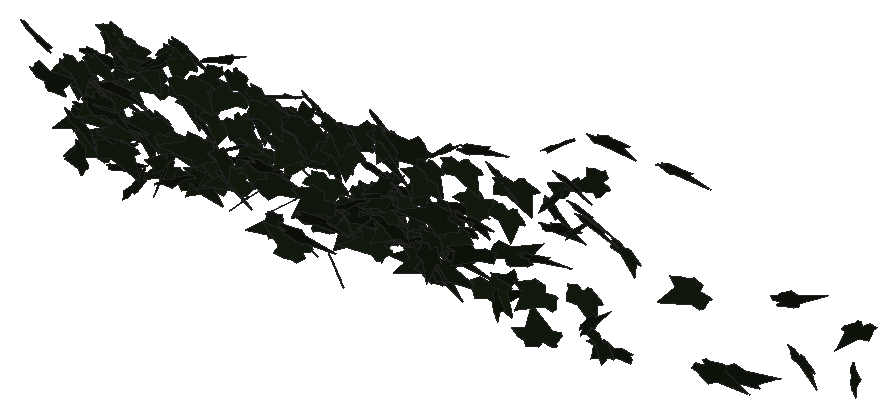
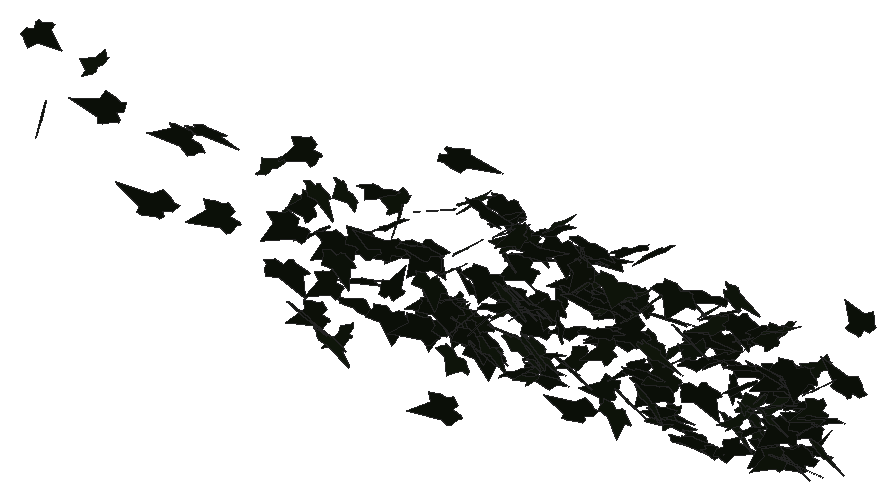
# SketchUp Ruby script. Lengths in millimetres.
U = 1.mm
M = Sketchup.active_model
def pt(a) = Geom::Point3d.new(a.map { |v| v * U })
def face(e, loops, mat)
  f = e.add_face(loops[0].map { |a| pt(a) })
  loops[1..].each { |l| e.add_face(l.map { |a| pt(a) }).erase! }
  f.material = f.back_material = mat if mat
  f
end
# faces: each face lists its corners as indices into pts; further lists are holes
def faces(e, pts, list, mat = nil) = list.each { |f| face(e, (f[0].is_a?(Array) ? f : [f]).map { |l| l.map { |i| pts[i] } }, mat) }
# xy, xz, yz: faces in a plane at the given z, y or x. An outline is a flat list of corners, or four numbers for a rectangle; further outlines are holes
def ring(l) = l.size == 4 ? [[l[0], l[1]], [l[2], l[1]], [l[2], l[3]], [l[0], l[3]]] : l.each_slice(2).to_a
def flat(e, list, mat, &to3) = list.each { |f| face(e, (f[0].is_a?(Array) ? f : [f]).map { |l| ring(l).map { |u, v| to3.(u, v) } }, mat) }
def xy(e, z, list, mat = nil) = flat(e, list, mat) { |x, y| [x, y, z] }
def xz(e, y, list, mat = nil) = flat(e, list, mat) { |x, z| [x, y, z] }
def yz(e, x, list, mat = nil) = flat(e, list, mat) { |y, z| [x, y, z] }
def lines(e, pts, list) = list.each { |a, b| e.add_line(pt(pts[a]), pt(pts[b])) }
# prism: a flat outline (further loops are holes) pulled along v
def prism(e, loops, v, mat = nil)
  f = face(e, loops, mat); d = Geom::Vector3d.new(v.map { |x| x * U })
  f.pushpull(f.normal.samedirection?(d) ? d.length : -d.length)
end
def box(e, o, s, mat = nil) = prism(e, [[o, [o[0] + s[0], o[1], o[2]], [o[0] + s[0], o[1] + s[1], o[2]], [o[0], o[1] + s[1], o[2]]]], [0, 0, s[2]], mat)
def at(x, y, z, deg = 0) = Geom::Transformation.translation(pt([x, y, z])) * Geom::Transformation.rotation(ORIGIN, Z_AXIS, deg.degrees)
def axes(o, x, y, z) = Geom::Transformation.new([*x, 0, *y, 0, *z, 0, *pt(o).to_a, 1])
def part(name) = M.definitions.add(name)
# library, detail: a bought-in or finely detailed component or shape, given as its bounding box
def library(name, o, s) = part(name).tap { |d| box(d.entities, o, s) }
def detail(e, o, s) = box(e.add_group.entities, o, s)
def put(e, d, t, mat = nil) = e.add_instance(d, t).tap { |i| i.material = mat if mat }
def group(e, t, mat = nil) = e.add_group.tap { |g| g.transformation = t; g.material = mat if mat }.entities
root = M.entities
M.materials.add("efeu1").color = [18, 25, 13]
c1 = part("ivyleaf_9")
p = [[39.1,54.8,31.7],[34.5,51.8,30.2],[-5.3,25.2,17.3],[-17.9,28.3,20.9],[-21.6,21.7,17],[-20.2,4.3,5.3],
  [-22.9,-0.3,2.5],[-17.1,-4,-0.6],[-2,-2.1,-1.2],[-0.7,-15.4,-10.1],[16.6,-22.3,-16.7],[21.1,-15.1,-12.5],
  [32.7,-10.7,-11],[46.1,-1.8,-6.6],[30.8,11.2,3.8]]
faces(c1.entities,p,[[0,1,2,3,4,5,6,7,8,9,10,11,12,13,14]],"efeu1")
put(root,c1,axes([6987.3,575.4,5164.4],[-1.35128,-1.10406,-0.33576],[0.69221,0.16003,-1.29534],[2.08434,-0.76891,0.21251]))
put(root,c1,axes([7044.1,521.7,5017.1],[-1.94294,0.95691,-0.16624],[0.20085,-0.13047,-1.39906],[-1.83753,-1.02607,0.02286]))
put(root,c1,axes([6987.6,400.2,5195.8],[-0.31285,0.13905,1.47625],[1.73968,-1.15999,0.21104],[2.22203,0.92777,0.04261]))
put(root,c1,axes([6992.9,326.4,5410.5],[-0.05139,-0.57991,1.37103],[1.05785,-1.27601,-0.52878],[2.62827,0.50224,0.23963]))
put(root,c1,axes([7007,583.9,5129],[0.31005,-1.35705,-0.09852],[-0.02649,0.09755,-1.36679],[2.5894,0.16349,-0.00219]))
put(root,c1,axes([6997.3,554.2,5179.8],[2.301,-0.69536,-0.09625],[-0.09394,0.10701,-1.39306],[1.33272,1.20811,0.06799]))
put(root,c1,axes([7043.8,504.4,5234.5],[-0.08437,-1.39838,0.16525],[-0.01937,-0.16501,-1.39908],[2.67985,-0.04522,-0.00491]))
put(root,c1,axes([7121.3,630.5,4983.1],[-2.28537,0.3892,0.4893],[-1.08791,-0.25428,-1.20059],[-0.48198,-1.27149,0.38988]))
put(root,c1,axes([7082.3,509.9,5078.4],[2.60564,0.29321,0.06626],[0.11968,0.0228,-1.4001],[-0.55946,1.3705,0.00911]))
put(root,c1,axes([7123.6,438.2,4916],[-0.35528,-0.20118,1.47783],[-1.22938,-1.33152,-0.26286],[2.55851,-0.66774,0.07891]))
put(root,c1,axes([7124.9,527.5,5287.4],[2.20419,0.45956,-0.79965],[-1.42967,-0.27475,-1.24586],[-1.01844,1.38031,0.01825]))
put(root,c1,axes([7153.9,497.5,4953.7],[-2.16775,-0.51688,0.6399],[-0.98134,-0.40294,-1.24328],[1.21979,-1.24275,0.13696]))
put(root,c1,axes([7096.2,619.4,5099.9],[2.58102,0.04148,-0.09359],[-0.17912,0.01609,-1.35665],[-0.07663,1.35928,0.01892]))
put(root,c1,axes([7107.5,520.1,5271.7],[1.0316,-1.16959,-0.59984],[-0.29748,0.58688,-1.28557],[2.48389,0.55604,0.09516]))
put(root,c1,axes([7149.5,508.2,5128.5],[-1.49282,-0.91359,0.64291],[-0.64363,-0.55451,-1.20057],[2.02635,-0.84917,0.0923]))
put(root,c1,axes([7168.1,558.9,4955.3],[-2.43955,0.46933,-0.21974],[0.37712,-0.09783,-1.36483],[-0.91134,-1.29683,0.02343]))
put(root,c1,axes([7090.1,540.8,4932.8],[0.54196,-0.25496,1.34292],[2.49688,-0.33411,-0.34163],[0.73031,1.3315,0.17142]))
put(root,c1,axes([7188.4,603.3,5117.5],[-1.42232,1.13045,0.23543],[-0.57317,0.07991,-1.33969],[-2.12158,-0.77945,0.2041]))
put(root,c1,axes([7120.3,626.1,4985.6],[2.35985,-0.43864,-0.32699],[-0.41444,0.34741,-1.29177],[0.95523,1.23437,0.24737]))
put(root,c1,axes([7145,596.4,5170.3],[1.45055,-1.13108,-0.30205],[0.0355,0.3721,-1.34635],[2.22782,0.73052,0.21812]))
put(root,c1,axes([7188.7,595.2,5147.3],[-1.44717,-1.12504,0.32421],[0.05347,-0.404,-1.33604],[2.22767,-0.72117,0.24268]))
put(root,c1,axes([7251.2,579.9,5274.8],[-2.61515,-0.03381,-0.1199],[0.23381,-0.14782,-1.36626],[0.03927,-1.37136,0.15023]))
put(root,c1,axes([7226.7,521.5,5401.1],[-1.51726,-0.92919,0.73564],[0.01191,-0.88988,-1.11723],[2.25553,-0.62036,0.50075]))
put(root,c1,axes([7189.6,489.2,5210.3],[2.76874,0.05186,0.25804],[0.49107,0.00505,-1.4557],[-0.09886,1.47748,-0.00409]))
put(root,c1,axes([7203.1,490.7,5399],[1.15331,-1.28618,-0.12622],[-0.07951,0.11984,-1.42172],[2.45833,0.60728,0.01323]))
put(root,c1,axes([7202.6,303.9,5157.4],[0.75456,-1.30208,0.61517],[0.46064,-0.56873,-1.35977],[2.70177,0.46061,0.06003]))
put(root,c1,axes([7201.2,411.6,5187.7],[-0.01399,-0.12223,-1.45499],[2.65777,0.42429,-0.0427],[0.81147,-1.39177,0.11476]))
put(root,c1,axes([7218.5,528.6,5381.5],[1.75038,-1.05899,0.26601],[0.27644,-0.22605,-1.4021],[2.05961,0.93033,-0.03788]))
put(root,c1,axes([7240.1,494.7,4909.3],[2.00993,0.74421,0.40226],[0.63052,0.22819,-1.29195],[-1.48144,1.10682,-0.00411]))
put(root,c1,axes([7252.6,584.9,5037.9],[-0.08734,-1.29505,-0.4348],[0.28474,0.42767,-1.28959],[2.58431,-0.09089,0.12739]))
put(root,c1,axes([7235.4,424,5135.1],[1.33394,-0.52509,1.12204],[1.82035,-0.58995,-0.87355],[1.49842,1.18414,0.06234]))
put(root,c1,axes([7280.5,491,5377.2],[0.04498,-1.06706,-1.07303],[-0.12078,1.07152,-1.06695],[2.87754,0.06165,-0.02801]))
put(root,c1,axes([7335.9,532.3,5056.2],[-1.16153,1.25574,0.27902],[-0.18578,0.26274,-1.39594],[-2.44115,-0.61749,-0.02653]))
put(root,c1,axes([7332.5,421.3,5106.3],[-0.90991,-0.47412,1.20223],[-1.56419,-0.87769,-0.67297],[1.89811,-0.95057,0.02174]))
put(root,c1,axes([7303.3,520.3,5101.6],[1.35793,-0.75192,-0.96683],[-0.88241,0.86984,-1.01865],[2.15758,0.82899,0.19189]))
put(root,c1,axes([7358,575.3,5238.1],[-2.17136,-0.2832,0.78427],[-1.1956,-0.58206,-1.12405],[1.04353,-1.25616,0.34404]))
put(root,c1,axes([7297.9,619.4,5065.5],[1.10209,-1.24001,-0.0136],[0.2012,0.06432,-1.36302],[2.35153,0.57565,0.123]))
put(root,c1,axes([7308.9,378.5,5059.4],[-0.94605,-0.56739,-1.25746],[2.0907,0.64572,-0.72562],[1.58822,-1.188,0.20617]))
put(root,c1,axes([7365.8,410.2,4886.1],[-1.30624,1.03083,-0.83423],[-0.99321,0.65359,1.23697],[2.3202,0.86013,0.05985]))
put(root,c1,axes([7326.4,511.8,5341],[0.0657,-1.43734,-0.0753],[0.59265,0.081,-1.40331],[2.67443,0.01736,0.31282]))
put(root,c1,axes([7343.6,509.1,5055],[-0.35681,-1.10272,0.87642],[0.44942,-0.89624,-1.07714],[2.64287,0.00353,0.30149]))
put(root,c1,axes([7392.4,585.4,4912.1],[-0.41198,-0.18922,-1.32688],[0.40946,-1.33155,0.15479],[-2.51779,-0.18558,0.24229]))
put(root,c1,axes([7407.9,497.9,5376.7],[0.42589,1.27383,-0.53827],[-0.07165,-0.53946,-1.2923],[-2.63094,0.2209,-0.05194]))
put(root,c1,axes([7426.8,515.5,4974],[-1.04629,1.19055,0.39748],[-0.30552,0.36368,-1.31134],[-2.36919,-0.57267,-0.00643]))
put(root,c1,axes([7391,501.5,5116.7],[-0.05299,-1.40594,-0.24864],[-0.03429,0.24901,-1.40603],[2.71708,-0.02427,-0.0226]))
put(root,c1,axes([7411.5,452.9,5162.2],[-1.55732,-0.68227,-0.87434],[1.59409,0.33202,-1.04295],[1.38348,-1.15056,0.21751]))
put(root,c1,axes([7404.6,599.3,5399.3],[1.86942,-0.96205,-0.2297],[0.12829,0.38808,-1.33715],[1.87806,0.93111,0.31998]))
put(root,c1,axes([7476.3,453.8,5439.4],[-1.74129,0.72344,-0.81171],[0.68212,-0.80089,-1.11779],[-1.95371,-0.92441,0.33319]))
put(root,c1,axes([7459.7,545.7,5395.9],[-0.83055,-1.35508,0.15136],[0.02238,-0.16266,-1.42233],[2.59494,-0.43231,0.06072]))
put(root,c1,axes([7533.7,557.8,5079.8],[0.24493,1.19937,-0.75286],[-0.55996,-0.71682,-1.19225],[-2.63628,0.26369,0.18329]))
put(root,c1,axes([7472.1,595.4,4906],[-0.28252,-0.47476,-1.3209],[2.29902,0.63324,-0.36335],[1.36046,-1.16869,0.33972]))
put(root,c1,axes([7511.1,595.5,5218.2],[-0.96129,-1.29081,-0.17502],[0.07123,0.17326,-1.38583],[2.47812,-0.5057,-0.02806]))
put(root,c1,axes([7519,395,5034.2],[-0.87839,0.45942,-1.23349],[1.69188,-0.85518,-0.65114],[-1.84748,-1.00158,-0.00983]))
put(root,c1,axes([7549.3,623,4908.6],[-2.37495,-0.53442,0.11195],[-0.19758,-0.04195,-1.35749],[1.02022,-1.25218,-0.0023]))
put(root,c1,axes([7527,407,5152.7],[0.42178,-1.04534,-0.88327],[-0.00579,0.8944,-1.05927],[2.6046,0.17126,0.14068]))
put(root,c1,axes([7551.3,447.9,5342.2],[0.33698,-1.42826,0.03133],[-0.02925,-0.03347,-1.43906],[2.71876,0.17667,-0.01937]))
put(root,c1,axes([7610.2,568,5286.8],[-2.27222,0.72043,-0.06653],[0.10954,-0.0334,-1.39442],[-1.3726,-1.19528,-0.00114]))
put(root,c1,axes([7614.3,622.8,4951.6],[-2.50126,-0.3388,0.11687],[-0.15696,-0.14642,-1.35182],[0.66379,-1.31128,0.12075]))
put(root,c1,axes([7575.5,523.6,5182.5],[0.60353,-1.16478,0.83285],[0.52107,-0.78797,-1.20626],[2.67492,0.4163,0.04706]))
put(root,c1,axes([7583,439,5380.6],[-0.49082,-0.96763,-0.97719],[1.34928,0.75838,-0.93807],[2.24271,-0.66803,0.35051]))
put(root,c1,axes([7617.8,561.2,5435.4],[1.49983,1.18306,0.22995],[0.03781,0.26195,-1.41582],[-2.29343,0.778,0.12703]))
put(root,c1,axes([7609.4,581.9,5173.5],[-0.72766,-1.23702,0.49471],[0.00106,-0.51483,-1.28689],[2.53559,-0.35479,0.14251]))
put(root,c1,axes([7663.6,493.3,5399.4],[-1.98425,0.98196,0.09227],[-0.13384,0.05992,-1.43221],[-1.87232,-1.04495,0.00459]))
put(root,c1,axes([7689.1,399,5157.3],[-1.81893,0.01019,1.01738],[-1.9363,0.00189,-0.95576],[-0.0159,-1.39587,0.00613]))
put(root,c1,axes([7666.6,255.1,5106.8],[0.75187,1.35802,-0.05307],[-0.03201,-0.05038,-1.41432],[-2.58637,0.39541,0.00208]))
put(root,c1,axes([7696.1,604.9,4957.4],[-2.09753,-0.34591,0.71878],[-1.32226,-0.18611,-1.15483],[0.74596,-1.30255,-0.02588]))
put(root,c1,axes([7621.7,590,4953.5],[1.7044,-1.06528,0.12002],[0.1563,-0.08776,-1.39168],[2.03427,0.89928,0.00637]))
put(root,c1,axes([7673.8,565.5,5318.7],[-2.41131,-0.65815,-0.08821],[0.51998,-0.34349,-1.36145],[1.15187,-1.22271,0.42994]))
put(root,c1,axes([7660.7,553.6,5089.7],[1.46282,0.64431,0.97009],[0.94644,0.86944,-0.97147],[-2.00417,0.88086,0.2493]))
put(root,c1,axes([7715.4,625.2,5022.3],[-0.8237,1.19139,0.5005],[-0.27125,0.4806,-1.26725],[-2.4444,-0.4548,-0.02803]))
put(root,c1,axes([7732.6,597.7,5196.1],[-1.76025,1.02033,-0.07781],[-0.47311,-0.32576,-1.31705],[-1.88919,-0.86911,0.40232]))
put(root,c1,axes([7684.3,584,5050.5],[2.28922,0.71154,0.09584],[0.14993,0.05507,-1.39751],[-1.35819,1.20538,0.00727]))
put(root,c1,axes([7696,557.9,5394.6],[1.03197,-1.19375,-0.50297],[-0.39952,0.45708,-1.31112],[2.43279,0.58144,-0.00196]))
put(root,c1,axes([7696.2,471.9,5136.2],[0.2715,-1.39849,0.51335],[0.02234,-0.51462,-1.40523],[2.83516,0.13797,-0.03809]))
put(root,c1,axes([7756.4,623.2,5099.4],[-2.48999,-0.40066,-0.0487],[0.09829,-0.00236,-1.36818],[0.76183,-1.30922,0.01737]))
put(root,c1,axes([7790.9,544.5,5082.6],[0.94105,-0.46832,-1.33611],[-0.38378,1.37753,-0.55746],[2.6671,0.36346,0.39121]))
put(root,c1,axes([7819.1,570.3,5347.1],[-0.62549,-1.25379,0.59137],[0.16826,-0.62548,-1.27698],[2.63295,-0.25788,0.22209]))
put(root,c1,axes([7816,556.4,5273.3],[-0.0783,-1.28781,0.54306],[-0.01946,-0.543,-1.28845],[2.65989,-0.04188,0.00656]))
put(root,c1,axes([7854.8,612.5,4907.1],[0.30768,1.31464,0.37443],[0.09376,0.37119,-1.32454],[-2.59984,0.16897,-0.00346]))
put(root,c1,axes([7830.9,477.9,5288.6],[0.88806,0.56571,1.22616],[1.12783,1.07992,-0.72375],[-2.30932,0.74496,0.11806]))
put(root,c1,axes([7888.2,348,5048],[0.44532,1.12059,0.81922],[0.41809,0.79041,-1.14393],[-2.60854,0.31799,-0.04349]))
put(root,c1,axes([7890.7,560.3,5376.3],[1.44978,1.16442,0.23272],[-0.64743,0.4789,-1.28267],[-2.16522,0.63647,0.53936]))
put(root,c1,axes([7923.9,504.3,4904.6],[-1.9309,0.86091,0.11384],[-0.19791,0.05336,-1.33033],[-1.64086,-1.01952,0.0265]))
put(root,c1,axes([7891.6,579.5,5319.4],[-1.87457,-0.72047,-0.66921],[1.09353,0.34699,-1.21923],[1.51874,-1.13912,0.05187]))
put(root,c1,axes([7882.4,609.9,5132],[2.11446,-0.81319,-0.04385],[-0.04755,0.0401,-1.3767],[1.54919,1.11114,0.01759]))
put(root,c1,axes([7877.8,461.7,5148.4],[2.72689,-0.13266,0.43871],[0.82904,-0.05363,-1.43886],[0.27125,1.49749,-0.01267]))
put(root,c1,axes([7901.9,307.4,5392.5],[0.87863,-1.10277,-0.88458],[-0.18529,0.90355,-1.17722],[2.68419,0.42335,0.20829]))
put(root,c1,axes([7891.2,575.5,5301.8],[-0.62176,-0.5384,-1.24007],[2.26776,0.48799,-0.52578],[1.21545,-1.1859,0.34664]))
put(root,c1,axes([7929.3,533.9,5266.2],[1.06011,-1.30764,-0.24104],[-0.13719,0.23126,-1.42113],[2.5269,0.56115,0.02397]))
put(root,c1,axes([7966.1,586.7,5173.8],[-1.92485,-0.96557,-0.03006],[0.04979,0.01613,-1.39827],[1.83789,-1.01169,0.0064]))
put(root,c1,axes([7931.4,453.8,5106.2],[0.58403,-0.21667,-1.432],[0.75115,1.4209,-0.13042],[2.65207,-0.35473,0.35229]))
put(root,c1,axes([7952.1,408,5424.7],[-0.16072,-1.33017,-0.49594],[0.26398,0.48671,-1.32903],[2.68889,-0.12729,0.10083]))
put(root,c1,axes([7954.9,514.7,4905.9],[1.70036,-0.95047,0.46252],[0.63948,-0.31882,-1.30421],[1.9074,0.95419,0.02494]))
put(root,c1,axes([8028.4,517.2,5355.2],[0.36726,0.87488,1.10872],[-0.1516,1.12398,-0.87306],[-2.68367,0.05624,0.20105]))
put(root,c1,axes([7975.3,647,4865.2],[0.04859,-0.00082,1.33622],[2.53634,0.09732,-0.0254],[-0.18516,1.33291,0.00268]))
put(root,c1,axes([8015.2,579.7,5397.7],[2.20869,-0.3505,-0.70777],[-1.28209,0.21742,-1.21224],[0.78469,1.34182,0.01154]))
put(root,c1,axes([8019.5,546.2,5326.1],[0.81052,-1.31597,-0.25207],[-0.21199,0.22881,-1.38272],[2.54126,0.43881,-0.03495]))
put(root,c1,axes([8026.5,585.4,5046.9],[1.98026,-0.90144,-0.2105],[-0.29327,0.1436,-1.37664],[1.73719,1.05181,0.00755]))
put(root,c1,axes([8092,398.8,5326.9],[-2.01482,-1.039,0.20658],[-0.24114,-0.16577,-1.48304],[2.00166,-1.0658,0.02928]))
put(root,c1,axes([8116.1,583.8,4994],[-2.37628,0.51279,-0.12514],[0.21256,-0.05745,-1.34973],[-0.98185,-1.25351,0.01067]))
put(root,c1,axes([8119.5,597.8,5128.5],[-0.0226,-0.19475,1.38092],[0.09637,1.38,0.19506],[-2.65242,0.0518,-0.00468]))
put(root,c1,axes([8105.9,562.5,5118.5],[-1.19925,-1.22041,-0.21851],[0.19118,0.19405,-1.37348],[2.35186,-0.63808,0.00023]))
put(root,c1,axes([8154.6,344.9,4957.8],[-1.85338,-1.02651,-0.21507],[-0.27081,-0.16146,1.41492],[-1.97761,0.98413,0.0078]))
put(root,c1,axes([8114.4,433.9,5394.6],[-2.07338,-0.34015,-0.8981],[1.619,0.28851,-1.14115],[0.84825,-1.38209,-0.01719]))
put(root,c1,axes([8158.1,648.6,4951.3],[-1.98903,-0.73248,-0.38309],[0.75955,0.09368,-1.26786],[1.37771,-1.10915,0.14591]))
put(root,c1,axes([8179,507.5,5402.2],[1.74598,0.3261,-1.05216],[-1.98869,-0.17571,-0.96554],[-0.66346,1.38484,0.12525]))
put(root,c1,axes([8177.4,623.4,5016.5],[-1.05245,-1.24059,-0.11508],[0.15281,0.09016,-1.35777],[2.3663,-0.5576,0.0365]))
put(root,c1,axes([8215.9,389.4,5158.8],[-2.61296,-0.36724,0.06682],[-0.12497,-0.01312,-1.42119],[0.69934,-1.37449,-0.00429]))
put(root,c1,axes([8239.1,430.3,5322.7],[-1.9581,-0.07722,0.93169],[-1.76882,-0.0655,-1.03174],[0.19261,-1.38647,-0.00315]))
put(root,c1,axes([8215.1,594.1,4946.6],[-2.42683,-0.3961,-0.03955],[0.07499,0.00649,-1.33522],[0.75388,-1.27573,0.00549]))
put(root,c1,axes([8225.9,604.9,5032.9],[-0.13604,1.14684,0.72913],[-0.48328,0.706,-1.13537],[-2.54089,-0.19569,0.17691]))
put(root,c1,axes([8234.9,606,5041.3],[-1.18674,1.20476,-0.05582],[-0.29542,-0.14248,-1.34126],[-2.27628,-0.60961,0.20317]))
put(root,c1,axes([8181.4,644.5,4953.6],[1.38322,-1.12236,-0.0183],[-0.02958,0.01174,-1.33711],[2.13616,0.72692,-0.00666]))
put(root,c1,axes([8258.2,413.9,5320.2],[-2.27933,0.68838,0.17548],[-0.33122,0.04919,-1.38068],[-1.31083,-1.20942,0.04373]))
put(root,c1,axes([8159.8,279.3,5060.2],[1.79045,-0.44332,1.00169],[1.75809,-0.38856,-1.03954],[1.12044,1.31811,0.03046]))
put(root,c1,axes([8213,461.9,5366.3],[-0.76163,-1.14474,-0.88651],[0.84366,0.77871,-1.20565],[2.62327,-0.5828,0.13036]))
put(root,c1,axes([8303.8,547.9,5350.7],[-0.86762,0.28225,1.35324],[-2.62776,-0.02329,-0.46027],[-0.12864,-1.42777,0.27502]))
put(root,c1,axes([8265.8,464.1,5127.8],[0.95752,1.28089,0.1585],[0.15292,0.13871,-1.37594],[-2.45161,0.50892,-0.02392]))
put(root,c1,axes([8243.9,445.2,5429.1],[-0.21847,-1.35787,0.53651],[0.0095,-0.53853,-1.3619],[2.77869,-0.10492,0.04684]))
put(root,c1,axes([8219.7,288.4,5138.2],[2.44475,-0.02055,0.63316],[1.20547,0.06786,-1.28281],[-0.02205,1.43051,0.06995]))
put(root,c1,axes([8304.4,614.6,5028.6],[-1.17499,1.18574,-0.03286],[-0.36067,-0.13516,-1.31682],[-2.22857,-0.60329,0.23044]))
put(root,c1,axes([8284.8,958.5,5118.5],[0.9088,0.96721,0.80847],[0.05387,0.85608,-1.04089],[-2.39857,0.3857,0.28295]))
put(root,c1,axes([8267.5,648.5,4934.2],[-0.58971,-1.29543,-0.06566],[-0.03126,0.07142,-1.33157],[2.46842,-0.30858,-0.03255]))
put(root,c1,axes([8267.1,538.7,5151.9],[1.2503,-1.07778,-0.75279],[-0.40675,0.74279,-1.24998],[2.46876,0.66822,0.1753]))
put(root,c1,axes([8254,513.2,5061.1],[1.89953,0.54618,-0.89303],[1.12367,0.7252,1.10339],[1.64518,-1.12594,0.27748]))
put(root,c1,axes([8297.2,415.2,5382.3],[-0.852,-1.43357,-0.10005],[0.05611,0.09561,-1.50184],[2.73443,-0.44864,-0.00035]))
put(root,c1,axes([8345.4,567.5,5143],[-2.27532,-0.67601,0.07235],[-0.06163,-0.08956,-1.37202],[1.29246,-1.19436,0.06194]))
put(root,c1,axes([8299,580.9,5432.2],[2.0341,-0.9039,-0.24977],[-0.42537,0.12227,-1.39886],[1.73334,1.09074,-0.05018]))
put(root,c1,axes([8372.7,533.2,5164.9],[-2.35594,0.59991,-0.12376],[0.18312,-0.08516,-1.37516],[-1.15131,-1.24114,0.03453]))
put(root,c1,axes([8301.9,967.9,4909.2],[2.03801,0.22816,0.82919],[1.51181,0.24505,-1.09327],[-0.62723,1.33199,0.0591]))
put(root,c1,axes([8401.5,535.2,5143.9],[-0.61977,0.33631,-1.32818],[-2.11832,-0.86102,0.05488],[-1.52056,1.06242,0.46491]))
put(root,c1,axes([8314.5,522.3,5272.5],[2.57126,-0.32608,-0.00191],[-0.00197,0.00383,-1.38981],[0.6206,1.35102,0.00348]))
put(root,c1,axes([8382.2,545.3,5168],[-2.05702,0.8425,-0.16461],[0.23128,-0.11184,-1.37033],[-1.6173,-1.08755,0.0134]))
put(root,c1,axes([8370.5,598.2,5036.3],[-2.55188,-0.32062,-0.13981],[0.4229,-0.35305,-1.32142],[0.5141,-1.30105,0.39303]))
put(root,c1,axes([8386.2,582.5,5190],[-1.38976,1.16159,0.10689],[-0.10185,0.09262,-1.37204],[-2.21774,-0.73217,-0.00397]))
put(root,c1,axes([8333.7,618.3,5132.8],[0.56409,-1.33638,-0.06778],[0.01669,0.07137,-1.36864],[2.54661,0.29555,0.02398]))
put(root,c1,axes([8405.6,627.5,4986.7],[-0.74268,1.27902,-0.09719],[0.0205,-0.09831,-1.33709],[-2.44115,-0.38995,0.01834]))
put(root,c1,axes([8369.4,273.5,4988.4],[0.08988,-0.43721,1.3925],[0.11491,-1.39145,-0.43893],[2.77539,0.07177,-0.02692]))
put(root,c1,axes([8393,606.8,5132.9],[-1.46875,-1.13212,-0.03722],[0.08667,0.01399,-1.36981],[2.15407,-0.7725,0.02973]))
put(root,c1,axes([8428.7,492.4,5255.1],[-1.87995,0.96189,-0.18111],[0.25157,-0.12386,-1.37875],[-1.84577,-0.99659,-0.00345]))
put(root,c1,axes([8396.5,537.7,5390.6],[-1.03094,-1.13622,0.61477],[-0.29712,-0.60416,-1.25418],[2.44068,-0.55349,0.107]))
put(root,c1,axes([8412.5,637.1,4963.6],[0.91813,1.21405,-0.3295],[-0.23752,-0.30497,-1.30638],[-2.38237,0.49829,0.00326]))
put(root,c1,axes([8384,542.6,5409.7],[0.15919,-1.39785,0.08215],[-0.0313,-0.08327,-1.40018],[2.66478,0.08253,-0.02136]))
put(root,c1,axes([8386.5,512.3,5343.9],[1.19001,-1.2148,0.28921],[0.40925,-0.21386,-1.36322],[2.34112,0.65488,0.0913]))
put(root,c1,axes([8434,654.8,4958.7],[-2.0866,-0.26636,-0.72385],[1.41235,-0.02137,-1.11614],[0.40014,-1.31359,0.16494]))
put(root,c1,axes([8452.3,640.7,5006.4],[1.3563,0.8805,-0.72368],[-0.85667,-0.56669,-1.13274],[-1.99282,0.84287,-0.00559]))
put(root,c1,axes([8409.3,954.6,5181],[1.91997,0.33998,0.83846],[1.4135,0.40602,-1.05823],[-0.98342,1.24734,0.11593]))
put(root,c1,axes([8452.3,565.1,5210.1],[1.80026,0.99244,-0.16489],[-0.21323,-0.121,-1.37101],[-1.90279,0.95252,-0.00236]))
put(root,c1,axes([8448.2,637.2,5042.6],[0.70828,-0.59504,-1.15024],[1.1374,-0.98283,0.70179],[-2.18658,-0.70399,-0.00753]))
put(root,c1,axes([8510.7,573.3,4952.5],[-1.71288,0.89881,0.43769],[-0.6728,0.26475,-1.27058],[-1.77973,-0.96513,0.05907]))
put(root,c1,axes([8492.2,595.9,5043.7],[1.11345,1.21298,-0.06639],[-0.27393,-0.00395,-1.34062],[-2.29571,0.58878,0.12777]))
put(root,c1,axes([8510.4,284.5,5227.4],[-1.08377,1.20528,-0.58163],[0.49361,-0.52072,-1.33299],[-2.49873,-0.62563,-0.01105]))
put(root,c1,axes([8543.3,496.5,5400.9],[-0.53273,0.4357,1.38305],[-1.8284,0.99937,-0.50926],[-2.06717,-0.99622,0.09402]))
put(root,c1,axes([8548.2,304.9,5133.6],[-1.71278,-0.31747,1.08852],[-1.77018,-0.58814,-0.94051],[1.23425,-1.28409,0.16165]))
put(root,c1,axes([8546.7,574,4949],[-2.49999,-0.20553,0.30416],[-0.56322,-0.0758,-1.32925],[0.4134,-1.34619,0.02841]))
put(root,c1,axes([8521.2,625.5,5031.8],[2.24737,0.30799,-0.57443],[-1.04964,-0.16135,-1.22025],[-0.6611,1.30319,-0.01532]))
put(root,c1,axes([8515.6,607.7,5037.4],[0.99461,-1.11443,-0.62384],[-0.57639,0.54669,-1.23031],[2.36136,0.60284,-0.03755]))
put(root,c1,axes([8518.1,594.2,5313.8],[0.453,-1.37389,-0.11875],[-0.00636,0.11993,-1.39425],[2.62453,0.23743,0.01712]))
put(root,c1,axes([8606,640.3,5075.1],[1.13432,0.91809,-0.79993],[-0.90409,-0.64474,-1.09392],[-2.13389,0.7612,0.03825]))
put(root,c1,axes([8637.5,537.9,4937],[-0.59917,0.56395,1.19527],[-1.18644,1.02008,-0.64549],[-2.21794,-0.69802,0.02239]))
put(root,c1,axes([8629.3,287.4,5247.3],[-1.30653,-1.02408,0.86523],[-0.98119,-0.69567,-1.23243],[2.35535,-0.85787,-0.03345]))
put(root,c1,axes([8619.6,622.5,5076],[-1.45939,-1.11957,0.1339],[0.13243,-0.20861,-1.34574],[2.14186,-0.74994,0.17444]))
put(root,c1,axes([8643.8,226.2,5281.5],[1.95816,0.12155,-1.068],[-2.0029,-0.18705,-1.03512],[-0.41645,1.47113,-0.04337]))
put(root,c1,axes([8625.3,585.4,5172.9],[-0.65992,-1.19087,0.54912],[-0.09711,-0.55531,-1.23651],[2.49391,-0.33674,0.09715]))
put(root,c1,axes([8638,492.2,5009.7],[1.76858,-0.61503,-0.92823],[-1.49411,0.49552,-1.11425],[1.50289,1.21639,-0.01542]))
put(root,c1,axes([8647.4,425.9,5371.8],[-1.33637,-0.99335,0.81584],[-0.15607,-0.89311,-1.15801],[2.44145,-0.60082,0.37254]))
put(root,c1,axes([8668,625,5141.8],[0.30683,1.35312,0.00386],[-0.01324,0.00472,-1.36267],[-2.57523,0.16119,0.00746]))
put(root,c1,axes([8643.1,453.9,5078],[-1.63756,0.19228,-1.18489],[2.16569,-0.3335,-0.88044],[-0.72738,-1.42585,0.04614]))
put(root,c1,axes([8624.9,516,4979],[1.33856,-1.23211,-0.24038],[-0.1198,0.24058,-1.41729],[2.38617,0.70326,0.06369]))
put(root,c1,axes([8668.9,620.5,4975.2],[0.78404,1.29916,0.1099],[0.03253,0.10986,-1.3628],[-2.48117,0.41197,0.01686]))
put(root,c1,axes([8625.9,497.4,4993.8],[0.24286,-0.14919,-1.46844],[1.48984,1.25639,-0.05962],[2.3815,-0.77077,0.18705]))
put(root,c1,axes([8649.3,373.1,5357.9],[1.06605,-1.27597,-0.4935],[-0.33789,0.46096,-1.39334],[2.58171,0.58721,0.02142]))
put(root,c1,axes([8664.2,552.8,5021.5],[2.46714,-0.13381,0.40419],[0.75633,-0.08464,-1.30254],[0.29084,1.35522,-0.04144]))
put(root,c1,axes([8685.5,565,5387.5],[-0.17974,-1.36865,-0.28529],[0.89317,0.23831,-1.29865],[2.50642,-0.18307,0.44232]))
put(root,c1,axes([8757.6,1077.9,5081.6],[-0.59504,1.26804,0.49947],[-0.73361,0.40925,-1.28027],[-2.4879,-0.42396,0.25805]))
put(root,c1,axes([8744.1,617.3,5242],[-2.10689,-0.75937,-0.27754],[0.47291,0.12824,-1.34201],[1.46426,-1.13406,0.03408]))
put(root,c1,axes([8725.2,559.5,5190.1],[2.52614,0.14047,-0.29244],[-0.56039,0.00441,-1.33428],[-0.25926,1.35914,0.03455]))
put(root,c1,axes([8740.6,989.3,5064.4],[1.79789,-0.96542,-0.37035],[-0.45534,0.28395,-1.35045],[1.91454,0.97413,0.02661]))
put(root,c1,axes([8804.7,965.2,5334.7],[0.00021,1.35101,-0.22901],[-0.01851,-0.229,-1.35098],[-2.60786,0.00173,0.00957]))
put(root,c1,axes([8834.9,458.7,5146.8],[0.82819,0.87156,-1.14125],[-0.97548,-1.01969,-0.97416],[-2.55297,0.67236,0.002]))
put(root,c1,axes([8886.2,232.3,5389.5],[-0.95828,-0.19864,-1.4024],[-1.74316,-1.08965,0.48319],[-2.05624,1.01632,0.24395]))
put(root,c1,axes([8815.5,605.3,5384.4],[1.01215,-1.13037,0.60093],[0.46216,-0.54984,-1.24915],[2.3922,0.58449,-0.01293]))
put(root,c1,axes([8861.7,595.5,4928.4],[1.225,1.16256,-0.35129],[-0.34482,-0.30121,-1.32879],[-2.28552,0.66856,0.01219]))
put(root,c1,axes([8895,1087.3,5157.9],[-2.34319,0.66709,0.14111],[-0.29697,0.00788,-1.39868],[-1.26326,-1.23922,0.06707]))
put(root,c1,axes([8831.7,950.4,5217.3],[2.4588,-0.4425,-0.15002],[-0.28448,0.02648,-1.36541],[0.84252,1.30034,-0.02324]))
put(root,c1,axes([8895.5,558,4981.9],[0.5684,0.37267,1.35675],[-1.74451,-1.00073,0.47665],[2.03158,-0.96359,0.0297]))
put(root,c1,axes([8886.1,577,5265.3],[-0.40009,-1.37384,0.06285],[-0.02096,-0.0619,-1.38983],[2.61735,-0.2105,-0.00152]))
put(root,c1,axes([8862.3,985.7,5097.2],[2.43258,-0.57149,0.1111],[0.19016,-0.04871,-1.40009],[1.09158,1.28205,-0.00367]))
put(root,c1,axes([8920.9,571.5,5389.5],[-0.99475,-0.90994,-0.91845],[1.26754,0.65961,-1.03251],[2.10902,-0.82562,0.18735]))
put(root,c1,axes([8923.8,530.9,5116.5],[-0.55682,-0.08966,1.44092],[2.73506,0.12258,0.29942],[-0.26289,1.46521,0.06312]))
put(root,c1,axes([8940.9,408.4,5075.3],[0.09046,-1.27417,-0.81821],[0.20297,0.81939,-1.26983],[2.87478,-0.01776,0.1154]))
put(root,c1,axes([8975.4,982.8,5408.3],[2.68712,0.21932,0.16636],[0.32182,-0.00502,-1.4285],[-0.4134,1.42165,-0.03071]))
put(root,c1,axes([9041.8,582,4994.4],[-2.12426,-0.75953,0.46039],[-0.42014,-0.47895,-1.32533],[1.63732,-1.10831,0.25722]))
put(root,c1,axes([8998.9,690.1,5197.5],[2.45309,0.42182,0.2362],[0.4281,0.0721,-1.3562],[-0.81444,1.30841,-0.00142]))
put(root,c1,axes([8995.4,550.4,5136.5],[2.18394,0.12093,0.76479],[1.3643,0.35092,-1.13106],[-0.55702,1.33362,0.22827]))
put(root,c1,axes([9059.4,595.7,5346.6],[-1.07666,0.91721,-0.8899],[-0.88479,0.75881,1.07763],[2.26558,0.73222,-0.00205]))
put(root,c1,axes([9080.1,526.1,4847.7],[-2.78577,0.17302,0.11325],[0.2125,-0.02018,1.4739],[0.33125,1.46797,0.00692]))
put(root,c1,axes([9085.2,260.9,5119.8],[0.77515,-0.21936,-1.35694],[-1.91617,0.91591,-0.45026],[1.78103,1.08087,0.10615]))
put(root,c1,axes([9202.1,586.1,5302.9],[-0.72661,1.35449,0.05648],[0.0031,0.05914,-1.40716],[-2.5801,-0.38138,-0.0176]))
put(root,c1,axes([9253,539.2,5088.9],[0.02609,-1.50693,-0.15959],[-0.01123,0.15954,-1.50698],[2.884,0.01425,-0.00442]))
put(root,c1,axes([9241.8,1023.6,5368.8],[2.6051,-0.08112,0.44483],[0.85249,0.04947,-1.3693],[0.11759,1.43842,0.07217]))
put(root,c1,axes([9277.6,516.4,5396.4],[2.53933,-0.45883,0.00894],[0.01585,-0.00327,-1.41093],[0.87326,1.33427,-0.00038]))
put(root,c1,axes([9378.2,540.8,4914.8],[1.06624,0.66093,-1.12253],[-1.62981,-0.73394,-0.85952],[-1.86821,1.01749,0.10917]))
put(root,c1,axes([9389.5,377.8,5068.7],[0.40658,0.32781,1.36881],[1.57498,1.09066,-0.39035],[-2.16686,0.85425,-0.02689]))
put(root,c1,axes([9411.5,568.3,5303.2],[0.08386,-1.23369,0.69336],[0.41786,-0.67934,-1.2227],[2.66077,0.14557,0.17017]))
put(root,c1,axes([9468.5,370.6,5043.9],[-0.26144,-1.06306,0.94263],[0.03345,-0.94823,-1.06681],[2.70385,-0.09106,0.10434]))
put(root,c1,axes([9786.6,502.5,5295.7],[-2.6468,-0.15246,0.37946],[-0.71169,-0.07034,-1.39876],[0.31503,-1.43983,0.02815]))
put(root,c1,axes([9901.9,571.7,4968.9],[0.33969,-0.29107,1.44721],[2.74255,-0.28194,-0.23443],[0.60958,1.43066,0.24824]))
put(root,c1,axes([9955.4,344.3,5127.9],[0.38899,-0.07819,-1.43977],[2.35959,0.75197,0.13516],[1.4011,-1.24469,0.1721]))
put(root,c1,axes([10073.2,616.7,5311.4],[0.94412,-0.06709,1.39867],[2.47589,0.57108,-0.434],[-0.98601,1.36975,0.24945]))
put(root,c1,axes([10345.3,370.6,5290.9],[0.71329,-1.30209,0.64596],[0.28982,-0.62825,-1.35473],[2.75111,0.40378,-0.02477]))
put(root,c1,axes([10437.3,545.1,5169.1],[0.62499,0.01191,-1.47112],[-2.14505,0.97081,-0.24373],[1.79954,1.15306,0.2204]))
put(root,c1,axes([10524.6,483.3,5423],[-0.15684,0.58545,-1.38828],[0.56091,-1.35724,-0.58985],[-2.81212,-0.30337,-0.04023]))
